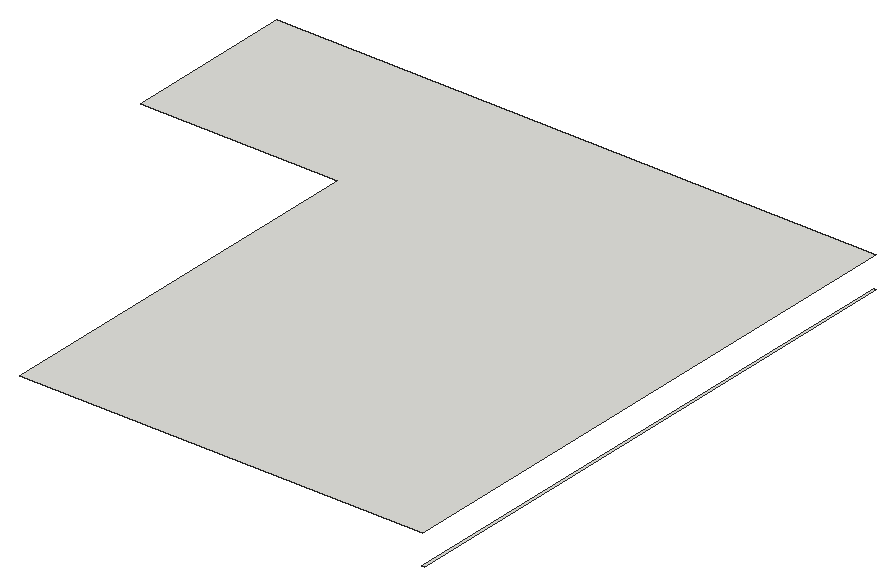
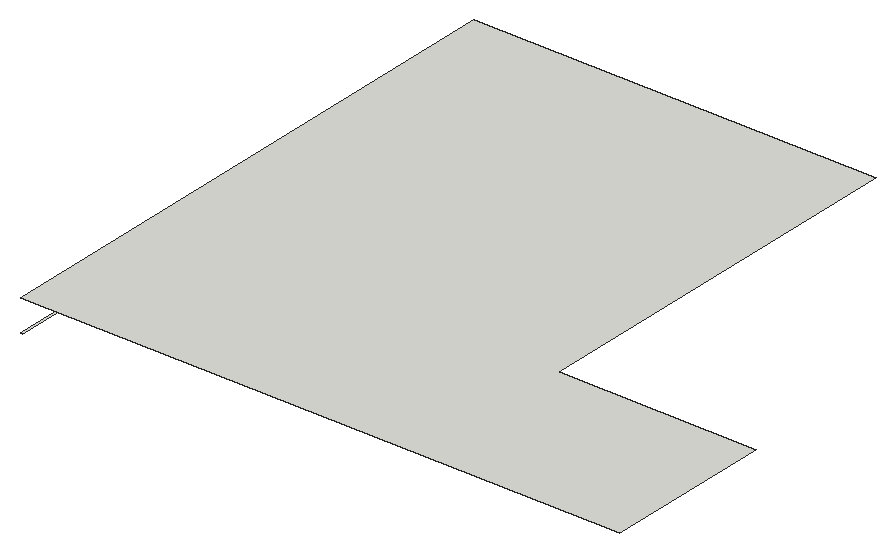
# SketchUp Ruby script. Lengths in inches.
U = 1.inch
M = Sketchup.active_model
def pt(a) = Geom::Point3d.new(a.map { |v| v * U })
def face(e, loops, mat)
  f = e.add_face(loops[0].map { |a| pt(a) })
  loops[1..].each { |l| e.add_face(l.map { |a| pt(a) }).erase! }
  f.material = f.back_material = mat if mat
  f
end
# faces: each face lists its corners as indices into pts; further lists are holes
def faces(e, pts, list, mat = nil) = list.each { |f| face(e, (f[0].is_a?(Array) ? f : [f]).map { |l| l.map { |i| pts[i] } }, mat) }
# xy, xz, yz: faces in a plane at the given z, y or x. An outline is a flat list of corners, or four numbers for a rectangle; further outlines are holes
def ring(l) = l.size == 4 ? [[l[0], l[1]], [l[2], l[1]], [l[2], l[3]], [l[0], l[3]]] : l.each_slice(2).to_a
def flat(e, list, mat, &to3) = list.each { |f| face(e, (f[0].is_a?(Array) ? f : [f]).map { |l| ring(l).map { |u, v| to3.(u, v) } }, mat) }
def xy(e, z, list, mat = nil) = flat(e, list, mat) { |x, y| [x, y, z] }
def xz(e, y, list, mat = nil) = flat(e, list, mat) { |x, z| [x, y, z] }
def yz(e, x, list, mat = nil) = flat(e, list, mat) { |y, z| [x, y, z] }
def lines(e, pts, list) = list.each { |a, b| e.add_line(pt(pts[a]), pt(pts[b])) }
# prism: a flat outline (further loops are holes) pulled along v
def prism(e, loops, v, mat = nil)
  f = face(e, loops, mat); d = Geom::Vector3d.new(v.map { |x| x * U })
  f.pushpull(f.normal.samedirection?(d) ? d.length : -d.length)
end
def box(e, o, s, mat = nil) = prism(e, [[o, [o[0] + s[0], o[1], o[2]], [o[0] + s[0], o[1] + s[1], o[2]], [o[0], o[1] + s[1], o[2]]]], [0, 0, s[2]], mat)
def at(x, y, z, deg = 0) = Geom::Transformation.translation(pt([x, y, z])) * Geom::Transformation.rotation(ORIGIN, Z_AXIS, deg.degrees)
def axes(o, x, y, z) = Geom::Transformation.new([*x, 0, *y, 0, *z, 0, *pt(o).to_a, 1])
def part(name) = M.definitions.add(name)
# library, detail: a bought-in or finely detailed component or shape, given as its bounding box
def library(name, o, s) = part(name).tap { |d| box(d.entities, o, s) }
def detail(e, o, s) = box(e.add_group.entities, o, s)
def put(e, d, t, mat = nil) = e.add_instance(d, t).tap { |i| i.material = mat if mat }
def group(e, t, mat = nil) = e.add_group.tap { |g| g.transformation = t; g.material = mat if mat }.entities
root = M.entities
xy(root,108.5,[[230,1,231,210]])
xy(root,110,[[156.34,21,156.26,21.01,156.1875,21.02,156.11,21.03,155.95,21.05,155.875,21.07,155.8,21.08,155.72,21.1,155.65,21.125,155.57,21.15,155.5,21.17,155.42,21.2,155.21,21.29,155.14,21.33,155.07,21.36,154.93,21.44,154.87,21.48,154.8,21.53,154.74,21.57,154.67,21.62,154.43,21.82,154.38,21.88,154.32,21.93,154.12,22.17,154.07,22.24,154.03,22.3,153.98,22.37,153.94,22.43,153.86,22.57,153.83,22.64,153.79,22.71,153.7,22.92,153.67,23,153.65,23.07,153.625,23.15,153.6,23.22,153.58,23.3,153.57,23.375,153.55,23.45,153.53,23.61,153.52,23.6875,153.51,23.76,153.5,23.84,153.5,24.16,153.51,24.24,153.52,24.3125,153.53,24.39,153.55,24.55,153.57,24.625,153.58,24.7,153.6,24.78,153.625,24.85,153.65,24.93,153.67,25,153.7,25.08,153.79,25.29,153.83,25.36,153.86,25.43,153.94,25.57,153.98,25.63,154.03,25.7,154.07,25.76,154.12,25.83,154.32,26.07,154.38,26.12,154.43,26.18,154.67,26.38,154.74,26.43,154.8,26.47,154.87,26.52,154.93,26.56,155.07,26.64,155.14,26.67,155.21,26.71,155.42,26.8,155.5,26.83,155.57,26.85,155.65,26.875,155.72,26.9,155.8,26.92,155.875,26.93,155.95,26.95,156.11,26.97,156.1875,26.98,156.26,26.99,156.34,27,156.66,27,156.74,26.99,156.8125,26.98,156.89,26.97,157.05,26.95,157.125,26.93,157.2,26.92,157.28,26.9,157.35,26.875,157.43,26.85,157.5,26.83,157.58,26.8,157.79,26.71,157.86,26.67,157.93,26.64,158.07,26.56,158.13,26.52,158.2,26.47,158.26,26.43,158.33,26.38,158.57,26.18,158.62,26.12,158.68,26.07,158.88,25.83,158.93,25.76,158.97,25.7,159.02,25.63,159.06,25.57,159.14,25.43,159.17,25.36,159.21,25.29,159.3,25.08,159.33,25,159.35,24.93,159.375,24.85,159.4,24.78,159.42,24.7,159.43,24.625,159.45,24.55,159.47,24.39,159.48,24.3125,159.49,24.24,159.5,24.16,159.5,23.84,159.49,23.76,159.48,23.6875,159.47,23.61,159.45,23.45,159.43,23.375,159.42,23.3,159.4,23.22,159.375,23.15,159.35,23.07,159.33,23,159.3,22.92,159.21,22.71,159.17,22.64,159.14,22.57,159.06,22.43,159.02,22.37,158.97,22.3,158.93,22.24,158.88,22.17,158.68,21.93,158.62,21.88,158.57,21.82,158.33,21.62,158.26,21.57,158.2,21.53,158.13,21.48,158.07,21.44,157.93,21.36,157.86,21.33,157.79,21.29,157.58,21.2,157.5,21.17,157.43,21.15,157.35,21.125,157.28,21.1,157.2,21.08,157.125,21.07,157.05,21.05,156.89,21.03,156.8125,21.02,156.74,21.01,156.66,21],[156.34,72.5,156.26,72.51,156.1875,72.52,156.11,72.53,155.95,72.55,155.875,72.57,155.8,72.58,155.72,72.6,155.65,72.625,155.57,72.65,155.5,72.67,155.42,72.7,155.21,72.79,155.14,72.83,155.07,72.86,154.93,72.94,154.87,72.98,154.8,73.03,154.74,73.07,154.67,73.12,154.43,73.32,154.38,73.38,154.32,73.43,154.12,73.67,154.07,73.74,154.03,73.8,153.98,73.87,153.94,73.93,153.86,74.07,153.83,74.14,153.79,74.21,153.7,74.42,153.67,74.5,153.65,74.57,153.625,74.65,153.6,74.72,153.58,74.8,153.57,74.875,153.55,74.95,153.53,75.11,153.52,75.1875,153.51,75.26,153.5,75.34,153.5,75.66,153.51,75.74,153.52,75.8125,153.53,75.89,153.55,76.05,153.57,76.125,153.58,76.2,153.6,76.28,153.625,76.35,153.65,76.43,153.67,76.5,153.7,76.58,153.79,76.79,153.83,76.86,153.86,76.93,153.94,77.07,153.98,77.13,154.03,77.2,154.07,77.26,154.12,77.33,154.32,77.57,154.38,77.62,154.43,77.68,154.67,77.88,154.74,77.93,154.8,77.97,154.87,78.02,154.93,78.06,155.07,78.14,155.14,78.17,155.21,78.21,155.42,78.3,155.5,78.33,155.57,78.35,155.65,78.375,155.72,78.4,155.8,78.42,155.875,78.43,155.95,78.45,156.11,78.47,156.1875,78.48,156.26,78.49,156.34,78.5,156.66,78.5,156.74,78.49,156.8125,78.48,156.89,78.47,157.05,78.45,157.125,78.43,157.2,78.42,157.28,78.4,157.35,78.375,157.43,78.35,157.5,78.33,157.58,78.3,157.79,78.21,157.86,78.17,157.93,78.14,158.07,78.06,158.13,78.02,158.2,77.97,158.26,77.93,158.33,77.88,158.57,77.68,158.62,77.62,158.68,77.57,158.88,77.33,158.93,77.26,158.97,77.2,159.02,77.13,159.06,77.07,159.14,76.93,159.17,76.86,159.21,76.79,159.3,76.58,159.33,76.5,159.35,76.43,159.375,76.35,159.4,76.28,159.42,76.2,159.43,76.125,159.45,76.05,159.47,75.89,159.48,75.8125,159.49,75.74,159.5,75.66,159.5,75.34,159.49,75.26,159.48,75.1875,159.47,75.11,159.45,74.95,159.43,74.875,159.42,74.8,159.4,74.72,159.375,74.65,159.35,74.57,159.33,74.5,159.3,74.42,159.21,74.21,159.17,74.14,159.14,74.07,159.06,73.93,159.02,73.87,158.97,73.8,158.93,73.74,158.88,73.67,158.68,73.43,158.62,73.38,158.57,73.32,158.33,73.12,158.26,73.07,158.2,73.03,158.13,72.98,158.07,72.94,157.93,72.86,157.86,72.83,157.79,72.79,157.58,72.7,157.5,72.67,157.43,72.65,157.35,72.625,157.28,72.6,157.2,72.58,157.125,72.57,157.05,72.55,156.89,72.53,156.8125,72.52,156.74,72.51,156.66,72.5],[156.34,124,156.26,124.01,156.1875,124.02,156.11,124.03,155.95,124.05,155.875,124.07,155.8,124.08,155.72,124.1,155.65,124.125,155.57,124.15,155.5,124.17,155.42,124.2,155.21,124.29,155.14,124.33,155.07,124.36,154.93,124.44,154.87,124.48,154.8,124.53,154.74,124.57,154.67,124.62,154.43,124.82,154.38,124.88,154.32,124.93,154.12,125.17,154.07,125.24,154.03,125.3,153.98,125.37,153.94,125.43,153.86,125.57,153.83,125.64,153.79,125.71,153.7,125.92,153.67,126,153.65,126.07,153.625,126.15,153.6,126.22,153.58,126.3,153.57,126.375,153.55,126.45,153.53,126.61,153.52,126.6875,153.51,126.76,153.5,126.84,153.5,127.16,153.51,127.24,153.52,127.3125,153.53,127.39,153.55,127.55,153.57,127.625,153.58,127.7,153.6,127.78,153.625,127.85,153.65,127.93,153.67,128,153.7,128.08,153.79,128.29,153.83,128.36,153.86,128.43,153.94,128.57,153.98,128.63,154.03,128.7,154.07,128.76,154.12,128.83,154.32,129.07,154.38,129.12,154.43,129.18,154.67,129.38,154.74,129.43,154.8,129.47,154.87,129.52,154.93,129.56,155.07,129.64,155.14,129.67,155.21,129.71,155.42,129.8,155.5,129.83,155.57,129.85,155.65,129.875,155.72,129.9,155.8,129.92,155.875,129.93,155.95,129.95,156.11,129.97,156.1875,129.98,156.26,129.99,156.34,130,156.66,130,156.74,129.99,156.8125,129.98,156.89,129.97,157.05,129.95,157.125,129.93,157.2,129.92,157.28,129.9,157.35,129.875,157.43,129.85,157.5,129.83,157.58,129.8,157.79,129.71,157.86,129.67,157.93,129.64,158.07,129.56,158.13,129.52,158.2,129.47,158.26,129.43,158.33,129.38,158.57,129.18,158.62,129.12,158.68,129.07,158.88,128.83,158.93,128.76,158.97,128.7,159.02,128.63,159.06,128.57,159.14,128.43,159.17,128.36,159.21,128.29,159.3,128.08,159.33,128,159.35,127.93,159.375,127.85,159.4,127.78,159.42,127.7,159.43,127.625,159.45,127.55,159.47,127.39,159.48,127.3125,159.49,127.24,159.5,127.16,159.5,126.84,159.49,126.76,159.48,126.6875,159.47,126.61,159.45,126.45,159.43,126.375,159.42,126.3,159.4,126.22,159.375,126.15,159.35,126.07,159.33,126,159.3,125.92,159.21,125.71,159.17,125.64,159.14,125.57,159.06,125.43,159.02,125.37,158.97,125.3,158.93,125.24,158.88,125.17,158.68,124.93,158.62,124.88,158.57,124.82,158.33,124.62,158.26,124.57,158.2,124.53,158.13,124.48,158.07,124.44,157.93,124.36,157.86,124.33,157.79,124.29,157.58,124.2,157.5,124.17,157.43,124.15,157.35,124.125,157.28,124.1,157.2,124.08,157.125,124.07,157.05,124.05,156.89,124.03,156.8125,124.02,156.74,124.01,156.66,124],[156.34,175.5,156.26,175.51,156.1875,175.52,156.11,175.53,155.95,175.55,155.875,175.57,155.8,175.58,155.72,175.6,155.65,175.625,155.57,175.65,155.5,175.67,155.42,175.7,155.21,175.79,155.14,175.83,155.07,175.86,154.93,175.94,154.87,175.98,154.8,176.03,154.74,176.07,154.67,176.12,154.43,176.32,154.38,176.38,154.32,176.43,154.12,176.67,154.07,176.74,154.03,176.8,153.98,176.87,153.94,176.93,153.86,177.07,153.83,177.14,153.79,177.21,153.7,177.42,153.67,177.5,153.65,177.57,153.625,177.65,153.6,177.72,153.58,177.8,153.57,177.875,153.55,177.95,153.53,178.11,153.52,178.1875,153.51,178.26,153.5,178.34,153.5,178.66,153.51,178.74,153.52,178.8125,153.53,178.89,153.55,179.05,153.57,179.125,153.58,179.2,153.6,179.28,153.625,179.35,153.65,179.43,153.67,179.5,153.7,179.58,153.79,179.79,153.83,179.86,153.86,179.93,153.94,180.07,153.98,180.13,154.03,180.2,154.07,180.26,154.12,180.33,154.32,180.57,154.38,180.62,154.43,180.68,154.67,180.88,154.74,180.93,154.8,180.97,154.87,181.02,154.93,181.06,155.07,181.14,155.14,181.17,155.21,181.21,155.42,181.3,155.5,181.33,155.57,181.35,155.65,181.375,155.72,181.4,155.8,181.42,155.875,181.43,155.95,181.45,156.11,181.47,156.1875,181.48,156.26,181.49,156.34,181.5,156.66,181.5,156.74,181.49,156.8125,181.48,156.89,181.47,157.05,181.45,157.125,181.43,157.2,181.42,157.28,181.4,157.35,181.375,157.43,181.35,157.5,181.33,157.58,181.3,157.79,181.21,157.86,181.17,157.93,181.14,158.07,181.06,158.13,181.02,158.2,180.97,158.26,180.93,158.33,180.88,158.57,180.68,158.62,180.62,158.68,180.57,158.88,180.33,158.93,180.26,158.97,180.2,159.02,180.13,159.06,180.07,159.14,179.93,159.17,179.86,159.21,179.79,159.3,179.58,159.33,179.5,159.35,179.43,159.375,179.35,159.4,179.28,159.42,179.2,159.43,179.125,159.45,179.05,159.47,178.89,159.48,178.8125,159.49,178.74,159.5,178.66,159.5,178.34,159.49,178.26,159.48,178.1875,159.47,178.11,159.45,177.95,159.43,177.875,159.42,177.8,159.4,177.72,159.375,177.65,159.35,177.57,159.33,177.5,159.3,177.42,159.21,177.21,159.17,177.14,159.14,177.07,159.06,176.93,159.02,176.87,158.97,176.8,158.93,176.74,158.88,176.67,158.68,176.43,158.62,176.38,158.57,176.32,158.33,176.12,158.26,176.07,158.2,176.03,158.13,175.98,158.07,175.94,157.93,175.86,157.86,175.83,157.79,175.79,157.58,175.7,157.5,175.67,157.43,175.65,157.35,175.625,157.28,175.6,157.2,175.58,157.125,175.57,157.05,175.55,156.89,175.53,156.8125,175.52,156.74,175.51,156.66,175.5]])
xy(root,120,[[82,0,231,0,231,210,9,210,9,147,82,147]])
xz(root,175.5,[[156.34,108,156.42,110],[156.42,108,156.5,110],[156.5,108,156.58,110],[156.58,108,156.66,110]])
xz(root,181.5,[[156.34,108,156.42,110],[156.42,108,156.5,110],[156.5,108,156.58,110],[156.58,108,156.66,110]])
yz(root,101.25,[[178.34,108,178.42,110],[178.42,108,178.5,110],[178.5,108,178.58,110],[178.58,108,178.66,110]])
yz(root,153.5,[[178.34,108,178.42,110],[178.42,108,178.5,110],[178.5,108,178.58,110],[178.58,108,178.66,110]])
yz(root,159.5,[[127,108,127.08,110],[127.08,108,127.16,110],[178.34,108,178.42,110],[178.42,108,178.5,110],[178.5,108,178.58,110],
  [178.58,108,178.66,110]])
p = [[159.48,127.3125,108],[159.49,127.24,108],[159.49,127.24,110],[159.48,127.3125,110],[159.5,127.16,108],[159.5,127.16,110],
  [159.47,127.39,108],[159.47,127.39,110],[159.46,127.47,108],[159.46,127.47,110],[159.43,127.625,108],[159.45,127.55,108],
  [159.45,127.55,110],[159.43,127.625,110],[159.42,127.7,108],[159.42,127.7,110],[159.4,127.78,108],[159.4,127.78,110],
  [159.375,127.85,108],[159.375,127.85,110],[159.33,128,108],[159.35,127.93,108],[159.35,127.93,110],[159.33,128,110],
  [159.3,128.08,108],[159.3,128.08,110],[159.24,128.22,108],[159.27,128.15,108],[159.27,128.15,110],[159.24,128.22,110],
  [159.21,128.29,108],[159.21,128.29,110],[159.17,128.36,108],[159.17,128.36,110],[159.1,128.5,108],[159.14,128.43,108],
  [159.14,128.43,110],[159.1,128.5,110],[159.06,128.57,108],[159.06,128.57,110],[158.97,128.7,108],[159.02,128.63,108],
  [159.02,128.63,110],[158.97,128.7,110],[158.93,128.76,108],[158.93,128.76,110],[158.83,128.89,108],[158.88,128.83,108],
  [158.88,128.83,110],[158.83,128.89,110],[158.78,128.95,108],[158.78,128.95,110],[156.03,175.54,108],[155.95,175.55,108],
  [155.95,175.55,110],[156.03,175.54,110],[156.11,175.53,108],[156.11,175.53,110],[156.1875,175.52,108],[156.1875,175.52,110],
  [156.26,175.51,108],[156.26,175.51,110],[156.34,175.5,108],[156.34,175.5,110],[156.74,175.51,108],[156.66,175.5,108],
  [156.66,175.5,110],[156.74,175.51,110],[156.8125,175.52,108],[156.8125,175.52,110],[156.89,175.53,108],[156.89,175.53,110],
  [156.97,175.54,108],[156.97,175.54,110],[157.05,175.55,108],[157.05,175.55,110],[98.875,175.57,108],[98.8,175.55,108],
  [98.8,175.55,110],[98.875,175.57,110],[98.95,175.58,108],[98.95,175.58,110],[99.03,175.6,108],[99.03,175.6,110],
  [99.1,175.625,108],[99.1,175.625,110],[99.18,175.65,108],[99.18,175.65,110],[99.25,175.67,108],[99.25,175.67,110],
  [155.57,175.65,108],[155.5,175.67,108],[155.5,175.67,110],[155.57,175.65,110],[155.65,175.625,108],[155.65,175.625,110],
  [155.72,175.6,108],[155.72,175.6,110],[155.8,175.58,108],[155.8,175.58,110],[155.875,175.57,108],[155.875,175.57,110],
  [157.125,175.57,108],[157.125,175.57,110],[157.2,175.58,108],[157.2,175.58,110],[157.28,175.6,108],[157.28,175.6,110],
  [157.35,175.625,108],[157.35,175.625,110],[157.43,175.65,108],[157.43,175.65,110],[157.5,175.67,108],[157.5,175.67,110],
  [99.33,175.7,108],[99.33,175.7,110],[99.4,175.73,108],[99.4,175.73,110],[99.47,175.76,108],[99.47,175.76,110],
  [155.35,175.73,108],[155.28,175.76,108],[155.28,175.76,110],[155.35,175.73,110],[155.42,175.7,108],[155.42,175.7,110],
  [157.58,175.7,108],[157.58,175.7,110],[157.65,175.73,108],[157.65,175.73,110],[157.72,175.76,108],[157.72,175.76,110],
  [99.54,175.79,108],[99.54,175.79,110],[99.61,175.83,108],[99.61,175.83,110],[99.68,175.86,108],[99.68,175.86,110],
  [155.14,175.83,108],[155.07,175.86,108],[155.07,175.86,110],[155.14,175.83,110],[155.21,175.79,108],[155.21,175.79,110],
  [157.79,175.79,108],[157.79,175.79,110],[157.86,175.83,108],[157.86,175.83,110],[157.93,175.86,108],[157.93,175.86,110],
  [99.75,175.9,108],[99.75,175.9,110],[99.82,175.94,108],[99.82,175.94,110],[99.88,175.98,108],[99.88,175.98,110],
  [154.93,175.94,108],[154.87,175.98,108],[154.87,175.98,110],[154.93,175.94,110],[155,175.9,108],[155,175.9,110],
  [158,175.9,108],[158,175.9,110],[158.07,175.94,108],[158.07,175.94,110],[158.13,175.98,108],[158.13,175.98,110],
  [99.95,176.03,108],[99.95,176.03,110],[100.01,176.07,108],[100.01,176.07,110],[154.8,176.03,108],[154.74,176.07,108],
  [154.74,176.07,110],[154.8,176.03,110],[158.2,176.03,108],[158.2,176.03,110],[158.26,176.07,108],[158.26,176.07,110],
  [100.08,176.12,108],[100.08,176.12,110],[100.14,176.17,108],[100.14,176.17,110],[154.67,176.12,108],[154.61,176.17,108],
  [154.61,176.17,110],[154.67,176.12,110],[158.33,176.12,108],[158.33,176.12,110],[158.39,176.17,108],[158.39,176.17,110],
  [100.2,176.22,108],[100.2,176.22,110],[100.26,176.27,108],[100.26,176.27,110],[154.55,176.22,108],[154.49,176.27,108],
  [154.49,176.27,110],[154.55,176.22,110],[158.45,176.22,108],[158.45,176.22,110],[158.51,176.27,108],[158.51,176.27,110],
  [100.32,176.32,108],[100.32,176.32,110],[100.37,176.38,108],[100.37,176.38,110],[154.43,176.32,108],[154.38,176.38,108],
  [154.38,176.38,110],[154.43,176.32,110],[158.57,176.32,108],[158.57,176.32,110],[158.62,176.38,108],[158.62,176.38,110],
  [100.43,176.43,108],[100.43,176.43,110],[100.48,176.49,108],[100.48,176.49,110],[154.32,176.43,108],[154.27,176.49,108],
  [154.27,176.49,110],[154.32,176.43,110],[158.68,176.43,108],[158.68,176.43,110],[158.73,176.49,108],[158.73,176.49,110],
  [100.53,176.55,108],[100.53,176.55,110],[154.22,176.55,108],[154.22,176.55,110],[158.78,176.55,108],[158.78,176.55,110],
  [100.58,176.61,108],[100.58,176.61,110],[100.63,176.67,108],[100.63,176.67,110],[154.17,176.61,108],[154.12,176.67,108],
  [154.12,176.67,110],[154.17,176.61,110],[158.83,176.61,108],[158.83,176.61,110],[158.88,176.67,108],[158.88,176.67,110],
  [100.68,176.74,108],[100.68,176.74,110],[100.72,176.8,108],[100.72,176.8,110],[154.07,176.74,108],[154.03,176.8,108],
  [154.03,176.8,110],[154.07,176.74,110],[158.93,176.74,108],[158.93,176.74,110],[158.97,176.8,108],[158.97,176.8,110],
  [100.77,176.87,108],[100.77,176.87,110],[153.98,176.87,108],[153.98,176.87,110],[159.02,176.87,108],[159.02,176.87,110],
  [100.81,176.93,108],[100.81,176.93,110],[100.85,177,108],[100.85,177,110],[153.94,176.93,108],[153.9,177,108],
  [153.9,177,110],[153.94,176.93,110],[159.06,176.93,108],[159.06,176.93,110],[159.1,177,108],[159.1,177,110],
  [100.89,177.07,108],[100.89,177.07,110],[153.86,177.07,108],[153.86,177.07,110],[159.14,177.07,108],[159.14,177.07,110],
  [100.92,177.14,108],[100.92,177.14,110],[100.96,177.21,108],[100.96,177.21,110],[153.83,177.14,108],[153.79,177.21,108],
  [153.79,177.21,110],[153.83,177.14,110],[159.17,177.14,108],[159.17,177.14,110],[159.21,177.21,108],[159.21,177.21,110],
  [100.99,177.28,108],[100.99,177.28,110],[153.76,177.28,108],[153.76,177.28,110],[159.24,177.28,108],[159.24,177.28,110],
  [101.02,177.35,108],[101.02,177.35,110],[153.73,177.35,108],[153.73,177.35,110],[159.27,177.35,108],[159.27,177.35,110],
  [101.05,177.42,108],[101.05,177.42,110],[101.08,177.5,108],[101.08,177.5,110],[153.7,177.42,108],[153.67,177.5,108],
  [153.67,177.5,110],[153.7,177.42,110],[159.3,177.42,108],[159.3,177.42,110],[159.33,177.5,108],[159.33,177.5,110],
  [101.1,177.57,108],[101.1,177.57,110],[153.65,177.57,108],[153.65,177.57,110],[159.35,177.57,108],[159.35,177.57,110],
  [101.125,177.65,108],[101.125,177.65,110],[101.15,177.72,108],[101.15,177.72,110],[153.625,177.65,108],[153.6,177.72,108],
  [153.6,177.72,110],[153.625,177.65,110],[159.375,177.65,108],[159.375,177.65,110],[159.4,177.72,108],[159.4,177.72,110],
  [101.17,177.8,108],[101.17,177.8,110],[153.58,177.8,108],[153.58,177.8,110],[159.42,177.8,108],[159.42,177.8,110],
  [101.18,177.875,108],[101.18,177.875,110],[153.57,177.875,108],[153.57,177.875,110],[159.43,177.875,108],[159.43,177.875,110],
  [101.2,177.95,108],[101.2,177.95,110],[153.55,177.95,108],[153.55,177.95,110],[159.45,177.95,108],[159.45,177.95,110],
  [101.21,178.03,108],[101.21,178.03,110],[101.22,178.11,108],[101.22,178.11,110],[153.54,178.03,108],[153.53,178.11,108],
  [153.53,178.11,110],[153.54,178.03,110],[159.46,178.03,108],[159.46,178.03,110],[159.47,178.11,108],[159.47,178.11,110],
  [101.23,178.1875,108],[101.23,178.1875,110],[153.52,178.1875,108],[153.52,178.1875,110],[159.48,178.1875,108],[159.48,178.1875,110],
  [101.24,178.26,108],[101.24,178.26,110],[153.51,178.26,108],[153.51,178.26,110],[159.49,178.26,108],[159.49,178.26,110],
  [101.25,178.34,108],[101.25,178.34,110],[153.5,178.34,108],[153.5,178.34,110],[159.5,178.34,108],[159.5,178.34,110],
  [101.23,178.8125,108],[101.24,178.74,108],[101.24,178.74,110],[101.23,178.8125,110],[101.25,178.66,108],[101.25,178.66,110],
  [153.5,178.66,108],[153.51,178.74,108],[153.51,178.74,110],[153.5,178.66,110],[153.52,178.8125,108],[153.52,178.8125,110],
  [159.48,178.8125,108],[159.49,178.74,108],[159.49,178.74,110],[159.48,178.8125,110],[159.5,178.66,108],[159.5,178.66,110],
  [101.22,178.89,108],[101.22,178.89,110],[153.53,178.89,108],[153.53,178.89,110],[159.47,178.89,108],[159.47,178.89,110],
  [101.21,178.97,108],[101.21,178.97,110],[153.54,178.97,108],[153.54,178.97,110],[159.46,178.97,108],[159.46,178.97,110],
  [101.18,179.125,108],[101.2,179.05,108],[101.2,179.05,110],[101.18,179.125,110],[153.55,179.05,108],[153.55,179.05,110],
  [153.57,179.125,108],[153.57,179.125,110],[159.43,179.125,108],[159.45,179.05,108],[159.45,179.05,110],[159.43,179.125,110],
  [101.17,179.2,108],[101.17,179.2,110],[153.58,179.2,108],[153.58,179.2,110],[159.42,179.2,108],[159.42,179.2,110],
  [101.15,179.28,108],[101.15,179.28,110],[153.6,179.28,108],[153.6,179.28,110],[159.4,179.28,108],[159.4,179.28,110],
  [101.125,179.35,108],[101.125,179.35,110],[153.625,179.35,108],[153.625,179.35,110],[159.375,179.35,108],[159.375,179.35,110],
  [101.08,179.5,108],[101.1,179.43,108],[101.1,179.43,110],[101.08,179.5,110],[153.65,179.43,108],[153.65,179.43,110],
  [153.67,179.5,108],[153.67,179.5,110],[159.33,179.5,108],[159.35,179.43,108],[159.35,179.43,110],[159.33,179.5,110],
  [101.05,179.58,108],[101.05,179.58,110],[153.7,179.58,108],[153.7,179.58,110],[159.3,179.58,108],[159.3,179.58,110],
  [100.99,179.72,108],[101.02,179.65,108],[101.02,179.65,110],[100.99,179.72,110],[153.73,179.65,108],[153.73,179.65,110],
  [153.76,179.72,108],[153.76,179.72,110],[159.24,179.72,108],[159.27,179.65,108],[159.27,179.65,110],[159.24,179.72,110],
  [100.96,179.79,108],[100.96,179.79,110],[153.79,179.79,108],[153.79,179.79,110],[159.21,179.79,108],[159.21,179.79,110],
  [100.92,179.86,108],[100.92,179.86,110],[153.83,179.86,108],[153.83,179.86,110],[159.17,179.86,108],[159.17,179.86,110],
  [100.85,180,108],[100.89,179.93,108],[100.89,179.93,110],[100.85,180,110],[153.86,179.93,108],[153.86,179.93,110],
  [153.9,180,108],[153.9,180,110],[159.1,180,108],[159.14,179.93,108],[159.14,179.93,110],[159.1,180,110],
  [100.81,180.07,108],[100.81,180.07,110],[153.94,180.07,108],[153.94,180.07,110],[159.06,180.07,108],[159.06,180.07,110],
  [100.72,180.2,108],[100.77,180.13,108],[100.77,180.13,110],[100.72,180.2,110],[153.98,180.13,108],[153.98,180.13,110],
  [154.03,180.2,108],[154.03,180.2,110],[158.97,180.2,108],[159.02,180.13,108],[159.02,180.13,110],[158.97,180.2,110],
  [100.68,180.26,108],[100.68,180.26,110],[154.07,180.26,108],[154.07,180.26,110],[158.93,180.26,108],[158.93,180.26,110],
  [100.58,180.39,108],[100.63,180.33,108],[100.63,180.33,110],[100.58,180.39,110],[154.12,180.33,108],[154.12,180.33,110],
  [154.17,180.39,108],[154.17,180.39,110],[158.83,180.39,108],[158.88,180.33,108],[158.88,180.33,110],[158.83,180.39,110],
  [100.48,180.51,108],[100.53,180.45,108],[100.53,180.45,110],[100.48,180.51,110],[154.22,180.45,108],[154.22,180.45,110],
  [154.27,180.51,108],[154.27,180.51,110],[158.73,180.51,108],[158.78,180.45,108],[158.78,180.45,110],[158.73,180.51,110],
  [100.43,180.57,108],[100.43,180.57,110],[154.32,180.57,108],[154.32,180.57,110],[158.68,180.57,108],[158.68,180.57,110],
  [100.32,180.68,108],[100.37,180.62,108],[100.37,180.62,110],[100.32,180.68,110],[154.38,180.62,108],[154.38,180.62,110],
  [154.43,180.68,108],[154.43,180.68,110],[158.57,180.68,108],[158.62,180.62,108],[158.62,180.62,110],[158.57,180.68,110],
  [100.2,180.78,108],[100.26,180.73,108],[100.26,180.73,110],[100.2,180.78,110],[154.49,180.73,108],[154.49,180.73,110],
  [154.55,180.78,108],[154.55,180.78,110],[158.45,180.78,108],[158.51,180.73,108],[158.51,180.73,110],[158.45,180.78,110],
  [100.08,180.88,108],[100.14,180.83,108],[100.14,180.83,110],[100.08,180.88,110],[154.61,180.83,108],[154.61,180.83,110],
  [154.67,180.88,108],[154.67,180.88,110],[158.33,180.88,108],[158.39,180.83,108],[158.39,180.83,110],[158.33,180.88,110],
  [99.95,180.97,108],[100.01,180.93,108],[100.01,180.93,110],[99.95,180.97,110],[154.74,180.93,108],[154.74,180.93,110],
  [154.8,180.97,108],[154.8,180.97,110],[158.2,180.97,108],[158.26,180.93,108],[158.26,180.93,110],[158.2,180.97,110],
  [99.82,181.06,108],[99.88,181.02,108],[99.88,181.02,110],[99.82,181.06,110],[154.87,181.02,108],[154.87,181.02,110],
  [154.93,181.06,108],[154.93,181.06,110],[158.07,181.06,108],[158.13,181.02,108],[158.13,181.02,110],[158.07,181.06,110],
  [99.61,181.17,108],[99.68,181.14,108],[99.68,181.14,110],[99.61,181.17,110],[99.75,181.1,108],[99.75,181.1,110],
  [155,181.1,108],[155,181.1,110],[155.07,181.14,108],[155.07,181.14,110],[155.14,181.17,108],[155.14,181.17,110],
  [157.86,181.17,108],[157.93,181.14,108],[157.93,181.14,110],[157.86,181.17,110],[158,181.1,108],[158,181.1,110],
  [99.4,181.27,108],[99.47,181.24,108],[99.47,181.24,110],[99.4,181.27,110],[99.54,181.21,108],[99.54,181.21,110],
  [155.21,181.21,108],[155.21,181.21,110],[155.28,181.24,108],[155.28,181.24,110],[155.35,181.27,108],[155.35,181.27,110],
  [157.65,181.27,108],[157.72,181.24,108],[157.72,181.24,110],[157.65,181.27,110],[157.79,181.21,108],[157.79,181.21,110],
  [99.18,181.35,108],[99.25,181.33,108],[99.25,181.33,110],[99.18,181.35,110],[99.33,181.3,108],[99.33,181.3,110],
  [155.42,181.3,108],[155.42,181.3,110],[155.5,181.33,108],[155.5,181.33,110],[155.57,181.35,108],[155.57,181.35,110],
  [157.43,181.35,108],[157.5,181.33,108],[157.5,181.33,110],[157.43,181.35,110],[157.58,181.3,108],[157.58,181.3,110],
  [98.875,181.43,108],[98.95,181.42,108],[98.95,181.42,110],[98.875,181.43,110],[99.03,181.4,108],[99.03,181.4,110],
  [99.1,181.375,108],[99.1,181.375,110],[155.65,181.375,108],[155.65,181.375,110],[155.72,181.4,108],[155.72,181.4,110],
  [155.8,181.42,108],[155.8,181.42,110],[155.875,181.43,108],[155.875,181.43,110],[155.95,181.45,108],[155.95,181.45,110],
  [156.03,181.46,108],[156.03,181.46,110],[156.97,181.46,108],[157.05,181.45,108],[157.05,181.45,110],[156.97,181.46,110],
  [157.125,181.43,108],[157.125,181.43,110],[157.2,181.42,108],[157.2,181.42,110],[157.28,181.4,108],[157.28,181.4,110],
  [157.35,181.375,108],[157.35,181.375,110],[156.11,181.47,108],[156.11,181.47,110],[156.1875,181.48,108],[156.1875,181.48,110],
  [156.26,181.49,108],[156.26,181.49,110],[156.34,181.5,108],[156.34,181.5,110],[156.66,181.5,108],[156.74,181.49,108],
  [156.74,181.49,110],[156.66,181.5,110],[156.8125,181.48,108],[156.8125,181.48,110],[156.89,181.47,108],[156.89,181.47,110]]
faces(root,p,[[0,1,2,3],[1,4,5,2],[6,0,3,7],[8,6,7,9],[10,11,12,13],[11,8,9,12],[14,10,13,15],[16,14,15,17],
  [18,16,17,19],[20,21,22,23],[21,18,19,22],[24,20,23,25],[26,27,28,29],[27,24,25,28],[30,26,29,31],[32,30,31,33],
  [34,35,36,37],[35,32,33,36],[38,34,37,39],[40,41,42,43],[41,38,39,42],[44,40,43,45],[46,47,48,49],[47,44,45,48],
  [50,46,49,51],[52,53,54,55],[56,52,55,57],[58,56,57,59],[60,58,59,61],[62,60,61,63],[64,65,66,67],[68,64,67,69],
  [70,68,69,71],[72,70,71,73],[74,72,73,75],[76,77,78,79],[80,76,79,81],[82,80,81,83],[84,82,83,85],[86,84,85,87],
  [88,86,87,89],[90,91,92,93],[94,90,93,95],[96,94,95,97],[98,96,97,99],[100,98,99,101],[53,100,101,54],[102,74,75,103],
  [104,102,103,105],[106,104,105,107],[108,106,107,109],[110,108,109,111],[112,110,111,113],[114,88,89,115],[116,114,115,117],[118,116,117,119],
  [120,121,122,123],[124,120,123,125],[91,124,125,92],[126,112,113,127],[128,126,127,129],[130,128,129,131],[132,118,119,133],[134,132,133,135],
  [136,134,135,137],[138,139,140,141],[142,138,141,143],[121,142,143,122],[144,130,131,145],[146,144,145,147],[148,146,147,149],[150,136,137,151],
  [152,150,151,153],[154,152,153,155],[156,157,158,159],[160,156,159,161],[139,160,161,140],[162,148,149,163],[164,162,163,165],[166,164,165,167],
  [168,154,155,169],[170,168,169,171],[172,173,174,175],[157,172,175,158],[176,166,167,177],[178,176,177,179],[180,170,171,181],[182,180,181,183],
  [184,185,186,187],[173,184,187,174],[188,178,179,189],[190,188,189,191],[192,182,183,193],[194,192,193,195],[196,197,198,199],[185,196,199,186],
  [200,190,191,201],[202,200,201,203],[204,194,195,205],[206,204,205,207],[208,209,210,211],[197,208,211,198],[212,202,203,213],[214,212,213,215],
  [216,206,207,217],[218,216,217,219],[220,221,222,223],[209,220,223,210],[224,214,215,225],[226,224,225,227],[228,218,219,229],[221,230,231,222],
  [232,226,227,233],[234,228,229,235],[236,234,235,237],[238,239,240,241],[230,238,241,231],[242,232,233,243],[244,242,243,245],[246,236,237,247],
  [248,246,247,249],[250,251,252,253],[239,250,253,240],[254,244,245,255],[256,254,255,257],[258,248,249,259],[251,260,261,252],[262,256,257,263],
  [264,258,259,265],[266,264,265,267],[268,269,270,271],[260,268,271,261],[272,262,263,273],[274,272,273,275],[276,266,267,277],[269,278,279,270],
  [280,274,275,281],[282,276,277,283],[284,282,283,285],[286,287,288,289],[278,286,289,279],[290,280,281,291],[292,290,291,293],[294,284,285,295],
  [287,296,297,288],[298,292,293,299],[300,294,295,301],[296,302,303,297],[304,298,299,305],[306,300,301,307],[308,306,307,309],[310,311,312,313],
  [302,310,313,303],[314,304,305,315],[316,314,315,317],[318,308,309,319],[311,320,321,312],[322,316,317,323],[324,318,319,325],[326,324,325,327],
  [328,329,330,331],[320,328,331,321],[332,322,323,333],[334,332,333,335],[336,326,327,337],[329,338,339,330],[340,334,335,341],[342,336,337,343],
  [338,344,345,339],[346,340,341,347],[348,342,343,349],[344,350,351,345],[352,346,347,353],[354,348,349,355],[356,354,355,357],[358,359,360,361],
  [350,358,361,351],[362,352,353,363],[364,362,363,365],[366,356,357,367],[359,368,369,360],[370,364,365,371],[372,366,367,373],[368,374,375,369],
  [376,370,371,377],[378,372,373,379],[374,380,381,375],[382,376,377,383],[384,385,386,387],[385,388,389,386],[390,391,392,393],[391,394,395,392],
  [396,397,398,399],[397,400,401,398],[402,384,387,403],[394,404,405,395],[406,396,399,407],[408,402,403,409],[404,410,411,405],[412,406,407,413],
  [414,415,416,417],[415,408,409,416],[410,418,419,411],[418,420,421,419],[422,423,424,425],[423,412,413,424],[426,414,417,427],[420,428,429,421],
  [430,422,425,431],[432,426,427,433],[428,434,435,429],[436,430,431,437],[438,432,433,439],[434,440,441,435],[442,436,437,443],[444,445,446,447],
  [445,438,439,446],[440,448,449,441],[448,450,451,449],[452,453,454,455],[453,442,443,454],[456,444,447,457],[450,458,459,451],[460,452,455,461],
  [462,463,464,465],[463,456,457,464],[458,466,467,459],[466,468,469,467],[470,471,472,473],[471,460,461,472],[474,462,465,475],[468,476,477,469],
  [478,470,473,479],[480,474,475,481],[476,482,483,477],[484,478,479,485],[486,487,488,489],[487,480,481,488],[482,490,491,483],[490,492,493,491],
  [494,495,496,497],[495,484,485,496],[498,486,489,499],[492,500,501,493],[502,494,497,503],[504,505,506,507],[505,498,499,506],[500,508,509,501],
  [508,510,511,509],[512,513,514,515],[513,502,503,514],[516,504,507,517],[510,518,519,511],[520,512,515,521],[522,523,524,525],[523,516,517,524],
  [518,526,527,519],[526,528,529,527],[530,531,532,533],[531,520,521,532],[534,535,536,537],[535,522,525,536],[528,538,539,529],[538,540,541,539],
  [542,543,544,545],[543,530,533,544],[546,534,537,547],[540,548,549,541],[550,542,545,551],[552,553,554,555],[553,546,547,554],[548,556,557,549],
  [556,558,559,557],[560,561,562,563],[561,550,551,562],[564,565,566,567],[565,552,555,566],[558,568,569,559],[568,570,571,569],[572,573,574,575],
  [573,560,563,574],[576,577,578,579],[577,564,567,578],[570,580,581,571],[580,582,583,581],[584,585,586,587],[585,572,575,586],[588,589,590,591],
  [589,576,579,590],[582,592,593,583],[592,594,595,593],[596,597,598,599],[597,584,587,598],[600,601,602,603],[601,588,591,602],[594,604,605,595],
  [604,606,607,605],[608,609,610,611],[609,596,599,610],[612,613,614,615],[613,616,617,614],[616,600,603,617],[606,618,619,607],[618,620,621,619],
  [620,622,623,621],[624,625,626,627],[625,628,629,626],[628,608,611,629],[630,631,632,633],[631,634,635,632],[634,612,615,635],[622,636,637,623],
  [636,638,639,637],[638,640,641,639],[642,643,644,645],[643,646,647,644],[646,624,627,647],[648,649,650,651],[649,652,653,650],[652,630,633,653],
  [640,654,655,641],[654,656,657,655],[656,658,659,657],[660,661,662,663],[661,664,665,662],[664,642,645,665],[666,667,668,669],[667,670,671,668],
  [670,672,673,671],[672,648,651,673],[658,674,675,659],[674,676,677,675],[676,678,679,677],[678,680,681,679],[680,682,683,681],[682,684,685,683],
  [686,687,688,689],[687,690,691,688],[690,692,693,691],[692,694,695,693],[694,696,697,695],[696,660,663,697],[684,698,699,685],[698,700,701,699],
  [700,702,703,701],[702,704,705,703],[706,707,708,709],[707,710,711,708],[710,712,713,711],[712,686,689,713]])
